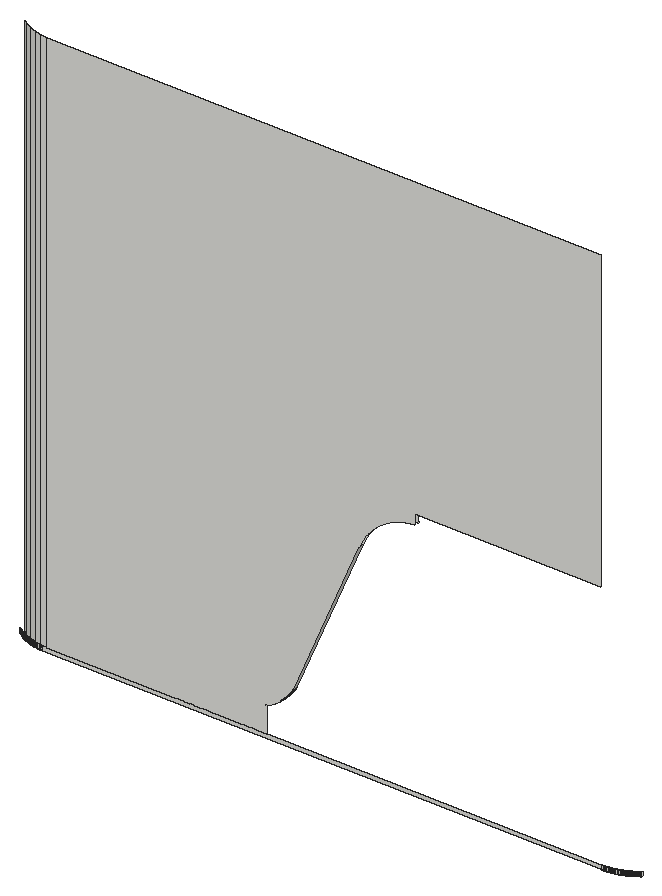
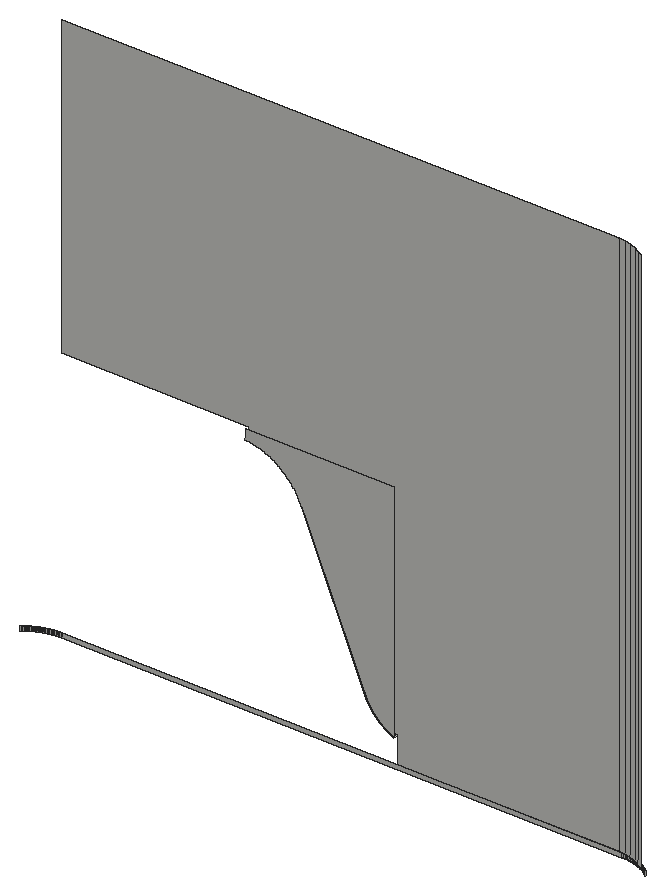
# SketchUp Ruby script. Lengths in inches.
U = 1.inch
M = Sketchup.active_model
def pt(a) = Geom::Point3d.new(a.map { |v| v * U })
def face(e, loops, mat)
  f = e.add_face(loops[0].map { |a| pt(a) })
  loops[1..].each { |l| e.add_face(l.map { |a| pt(a) }).erase! }
  f.material = f.back_material = mat if mat
  f
end
# faces: each face lists its corners as indices into pts; further lists are holes
def faces(e, pts, list, mat = nil) = list.each { |f| face(e, (f[0].is_a?(Array) ? f : [f]).map { |l| l.map { |i| pts[i] } }, mat) }
# xy, xz, yz: faces in a plane at the given z, y or x. An outline is a flat list of corners, or four numbers for a rectangle; further outlines are holes
def ring(l) = l.size == 4 ? [[l[0], l[1]], [l[2], l[1]], [l[2], l[3]], [l[0], l[3]]] : l.each_slice(2).to_a
def flat(e, list, mat, &to3) = list.each { |f| face(e, (f[0].is_a?(Array) ? f : [f]).map { |l| ring(l).map { |u, v| to3.(u, v) } }, mat) }
def xy(e, z, list, mat = nil) = flat(e, list, mat) { |x, y| [x, y, z] }
def xz(e, y, list, mat = nil) = flat(e, list, mat) { |x, z| [x, y, z] }
def yz(e, x, list, mat = nil) = flat(e, list, mat) { |y, z| [x, y, z] }
def lines(e, pts, list) = list.each { |a, b| e.add_line(pt(pts[a]), pt(pts[b])) }
# prism: a flat outline (further loops are holes) pulled along v
def prism(e, loops, v, mat = nil)
  f = face(e, loops, mat); d = Geom::Vector3d.new(v.map { |x| x * U })
  f.pushpull(f.normal.samedirection?(d) ? d.length : -d.length)
end
def box(e, o, s, mat = nil) = prism(e, [[o, [o[0] + s[0], o[1], o[2]], [o[0] + s[0], o[1] + s[1], o[2]], [o[0], o[1] + s[1], o[2]]]], [0, 0, s[2]], mat)
def at(x, y, z, deg = 0) = Geom::Transformation.translation(pt([x, y, z])) * Geom::Transformation.rotation(ORIGIN, Z_AXIS, deg.degrees)
def axes(o, x, y, z) = Geom::Transformation.new([*x, 0, *y, 0, *z, 0, *pt(o).to_a, 1])
def part(name) = M.definitions.add(name)
# library, detail: a bought-in or finely detailed component or shape, given as its bounding box
def library(name, o, s) = part(name).tap { |d| box(d.entities, o, s) }
def detail(e, o, s) = box(e.add_group.entities, o, s)
def put(e, d, t, mat = nil) = e.add_instance(d, t).tap { |i| i.material = mat if mat }
def group(e, t, mat = nil) = e.add_group.tap { |g| g.transformation = t; g.material = mat if mat }.entities
root = M.entities
xz(root,144,[[23.87,130,24.1875,132],[24.1875,130,290.26,132],[290.26,130,290.58,132],[26,132,131,132,131,144.27,130.48,144.04,131,144.28,131.27,144.38,131.36,144.43,131.53,144.5,131.79,144.63,132.04,144.75,132.56,145.01,132.8125,145.14,133.0625,145.28,133.32,145.42,133.57,145.56,133.81,145.7,134.0625,145.85,134.31,146,134.79,146.3,135.04,146.46,135.27,146.61,135.51,146.77,135.75,146.9375,135.98,147.1,136.22,147.27,136.68,147.61,136.9,147.79,137.13,147.97,137.35,148.15,137.58,148.33,137.8,148.51,138.01,148.7,138.23,148.89,138.44,149.08,138.66,149.27,138.87,149.47,139.08,149.66,139.28,149.86,139.49,150.0625,139.6875,150.27,139.89,150.47,140.09,150.68,140.28,150.89,140.48,151.1,140.67,151.32,140.86,151.53,141.05,151.75,141.23,151.97,141.41,152.1875,141.59,152.41,141.77,152.64,141.95,152.86,142.29,153.32,142.46,153.56,142.63,153.79,142.79,154.02,143.27,154.74,143.42,154.98,143.58,155.23,143.73,155.47,175.01,227.16,175.15,227.49,175.3,227.82,175.44,228.14,175.59,228.47,175.74,228.79,175.9,229.11,176.06,229.42,176.22,229.74,176.39,230.05,176.5625,230.36,176.74,230.67,177.1,231.29,177.28,231.59,177.66,232.19,177.86,232.49,178.26,233.07,178.68,233.65,178.89,233.9375,179.1,234.22,179.32,234.5,179.55,234.78,179.77,235.05,180,235.33,180.23,235.6,180.46,235.86,180.7,236.13,180.94,236.39,181.1875,236.65,181.43,236.9,181.68,237.16,181.93,237.41,182.19,237.66,182.97,238.38,183.24,238.62,184.05,239.31,184.89,239.97,185.18,240.18,185.46,240.39,185.75,240.6,186.04,240.8,186.34,241,186.63,241.2,187.23,241.58,187.54,241.77,187.84,241.95,188.46,242.31,189.08,242.65,189.4,242.8125,189.71,242.97,190.35,243.29,190.67,243.4375,191,243.58,191.32,243.73,191.65,243.87,192.97,244.39,193.31,244.51,193.64,244.625,193.98,244.74,194.32,244.85,195.34,245.15,195.68,245.24,196.03,245.33,196.375,245.42,196.72,245.5,197.07,245.58,197.42,245.65,197.76,245.72,198.11,245.78,198.46,245.85,198.81,245.9,199.17,245.96,199.52,246.01,200.22,246.09,200.58,246.13,200.93,246.16,201.29,246.19,201.64,246.22,201.56,248,201.56,251,290.45,251,290.45,392.81,26,392.81],[130.48,144.04,131,144.27,131,144.28]])
xz(root,146,[[131,144.28,131,251,201.56,251,201.56,248,201.64,246.22,201.29,246.19,200.93,246.16,200.58,246.13,200.22,246.09,199.52,246.01,199.17,245.96,198.81,245.9,198.46,245.85,198.11,245.78,197.76,245.72,197.42,245.65,197.07,245.58,196.72,245.5,196.375,245.42,196.03,245.33,195.68,245.24,195.34,245.15,194.32,244.85,193.98,244.74,193.64,244.625,193.31,244.51,192.97,244.39,191.65,243.87,191.32,243.73,191,243.58,190.67,243.4375,190.35,243.29,189.71,242.97,189.4,242.8125,189.08,242.65,188.46,242.31,187.84,241.95,187.54,241.77,187.23,241.58,186.63,241.2,186.34,241,186.04,240.8,185.75,240.6,185.46,240.39,185.18,240.18,184.89,239.97,184.05,239.31,183.24,238.62,182.97,238.38,182.19,237.66,181.93,237.41,181.68,237.16,181.43,236.9,181.1875,236.65,180.94,236.39,180.7,236.13,180.46,235.86,180.23,235.6,180,235.33,179.77,235.05,179.55,234.78,179.32,234.5,179.1,234.22,178.89,233.9375,178.68,233.65,178.26,233.07,177.86,232.49,177.66,232.19,177.28,231.59,177.1,231.29,176.74,230.67,176.5625,230.36,176.39,230.05,176.22,229.74,176.06,229.42,175.9,229.11,175.74,228.79,175.59,228.47,175.44,228.14,175.3,227.82,175.15,227.49,175.01,227.16,143.73,155.47,143.58,155.23,143.42,154.98,143.27,154.74,142.79,154.02,142.63,153.79,142.46,153.56,142.29,153.32,141.95,152.86,141.77,152.64,141.59,152.41,141.41,152.1875,141.23,151.97,141.05,151.75,140.86,151.53,140.67,151.32,140.48,151.1,140.28,150.89,140.09,150.68,139.89,150.47,139.6875,150.27,139.49,150.0625,139.28,149.86,139.08,149.66,138.87,149.47,138.66,149.27,138.44,149.08,138.23,148.89,138.01,148.7,137.8,148.51,137.58,148.33,137.35,148.15,137.13,147.97,136.9,147.79,136.68,147.61,136.22,147.27,135.98,147.1,135.75,146.9375,135.51,146.77,135.27,146.61,135.04,146.46,134.79,146.3,134.31,146,134.0625,145.85,133.81,145.7,133.57,145.56,133.32,145.42,133.0625,145.28,132.8125,145.14,132.56,145.01,132.04,144.75,131.79,144.63,131.53,144.5,131.36,144.43,131.27,144.38]])
p = [[22.61,144.05,130],[22.92,144.03,130],[22.92,144.03,132],[22.61,144.05,132],[23.24,144.02,130],[23.24,144.02,132],
  [23.56,144.01,130],[23.56,144.01,132],[23.87,144,130],[23.87,144,132],[290.58,144,130],[290.9,144.01,130],
  [290.9,144.01,132],[290.58,144,132],[291.21,144.02,130],[291.21,144.02,132],[291.53,144.03,130],[291.53,144.03,132],
  [291.85,144.05,130],[291.85,144.05,132],[21.35,144.17,130],[21.66,144.13,130],[21.66,144.13,132],[21.35,144.17,132],
  [21.98,144.1,130],[21.98,144.1,132],[22.29,144.07,130],[22.29,144.07,132],[292.16,144.07,130],[292.16,144.07,132],
  [292.48,144.1,130],[292.48,144.1,132],[292.79,144.13,130],[292.79,144.13,132],[293.11,144.17,130],[293.11,144.17,132],
  [20.4,144.3,130],[20.72,144.25,130],[20.72,144.25,132],[20.4,144.3,132],[21.03,144.21,130],[21.03,144.21,132],
  [293.42,144.21,130],[293.42,144.21,132],[293.74,144.25,130],[293.74,144.25,132],[294.05,144.3,130],[294.05,144.3,132],
  [19.78,144.4,130],[20.09,144.35,130],[20.09,144.35,132],[19.78,144.4,132],[294.36,144.35,130],[294.36,144.35,132],
  [294.67,144.4,130],[294.67,144.4,132],[19.47,144.46,130],[19.47,144.46,132],[294.98,144.46,130],[294.98,144.46,132],
  [18.85,144.59,130],[19.16,144.52,130],[19.16,144.52,132],[18.85,144.59,132],[295.29,144.52,130],[295.29,144.52,132],
  [295.6,144.59,130],[295.6,144.59,132],[18.54,144.66,130],[18.54,144.66,132],[295.91,144.66,130],[295.91,144.66,132],
  [17.93,144.82,130],[18.23,144.74,130],[18.23,144.74,132],[17.93,144.82,132],[296.22,144.74,130],[296.22,144.74,132],
  [296.53,144.82,130],[296.53,144.82,132],[17.62,144.9,130],[17.62,144.9,132],[296.83,144.9,130],[296.83,144.9,132],
  [17.32,144.99,130],[17.32,144.99,132],[297.13,144.99,130],[297.13,144.99,132],[17.02,145.08,130],[17.02,145.08,132],
  [297.4375,145.08,130],[297.4375,145.08,132],[16.71,145.17,130],[16.71,145.17,132],[297.74,145.17,130],[297.74,145.17,132],
  [16.41,145.27,130],[16.41,145.27,132],[298.04,145.27,130],[298.04,145.27,132],[16.11,145.375,130],[16.11,145.375,132],
  [298.34,145.375,130],[298.34,145.375,132],[15.82,145.48,130],[15.82,145.48,132],[298.64,145.48,130],[298.64,145.48,132],
  [15.52,145.59,130],[15.52,145.59,132],[298.93,145.59,130],[298.93,145.59,132],[15.23,145.71,130],[15.23,145.71,132],
  [299.23,145.71,130],[299.23,145.71,132],[14.93,145.83,130],[14.93,145.83,132],[299.52,145.83,130],[299.52,145.83,132],
  [14.64,145.95,130],[14.64,145.95,132],[299.8125,145.95,130],[299.8125,145.95,132],[14.35,146.07,130],[14.35,146.07,132],
  [300.1,146.07,130],[300.1,146.07,132],[14.0625,146.2,130],[14.0625,146.2,132],[300.39,146.2,130],[300.39,146.2,132],
  [13.78,146.34,130],[13.78,146.34,132],[300.68,146.34,130],[300.68,146.34,132],[13.49,146.48,130],[13.49,146.48,132],
  [300.96,146.48,130],[300.96,146.48,132],[13.21,146.62,130],[13.21,146.62,132],[301.25,146.62,130],[301.25,146.62,132],
  [12.93,146.76,130],[12.93,146.76,132],[301.53,146.76,130],[301.53,146.76,132],[12.65,146.91,130],[12.65,146.91,132],
  [301.81,146.91,130],[301.81,146.91,132],[12.37,147.06,130],[12.37,147.06,132],[302.08,147.06,130],[302.08,147.06,132],
  [12.09,147.22,130],[12.09,147.22,132],[302.36,147.22,130],[302.36,147.22,132],[11.82,147.375,130],[11.82,147.375,132],
  [302.63,147.375,130],[302.63,147.375,132],[11.55,147.54,130],[11.55,147.54,132],[302.9,147.54,130],[302.9,147.54,132],
  [11.28,147.7,130],[11.28,147.7,132],[303.17,147.7,130],[303.17,147.7,132],[11.01,147.87,130],[11.01,147.87,132],
  [303.4375,147.87,130],[303.4375,147.87,132],[10.75,148.04,130],[10.75,148.04,132],[303.7,148.04,130],[303.7,148.04,132],
  [10.49,148.22,130],[10.49,148.22,132],[303.97,148.22,130],[303.97,148.22,132],[10.23,148.4,130],[10.23,148.4,132],
  [304.23,148.4,130],[304.23,148.4,132],[9.97,148.58,130],[9.97,148.58,132],[304.48,148.58,130],[304.48,148.58,132],
  [9.72,148.77,130],[9.72,148.77,132],[304.74,148.77,130],[304.74,148.77,132],[9.46,148.96,130],[9.46,148.96,132],
  [304.99,148.96,130],[304.99,148.96,132],[9.21,149.15,130],[9.21,149.15,132],[305.24,149.15,130],[305.24,149.15,132],
  [8.97,149.35,130],[8.97,149.35,132],[305.49,149.35,130],[305.49,149.35,132],[8.72,149.55,130],[8.72,149.55,132],
  [305.73,149.55,130],[305.73,149.55,132],[22.87,144.21,132],[26,144,132],[26,144,392.81],[22.87,144.21,392.81],
  [19.79,144.82,132],[19.79,144.82,392.81],[16.82,145.83,132],[16.82,145.83,392.81],[14,147.22,132],[14,147.22,392.81],
  [11.39,148.96,132],[11.39,148.96,392.81],[131.27,144,144.38],[131,144,144.28],[131,146,144.28],[131.27,146,144.38],
  [131.36,144,144.43],[131.36,146,144.43],[131.53,144,144.5],[131.53,146,144.5],[131.79,144,144.63],[131.79,146,144.63],
  [132.04,144,144.75],[132.04,146,144.75],[132.3,144,144.88],[132.3,146,144.88],[132.56,144,145.01],[132.56,146,145.01],
  [132.8125,144,145.14],[132.8125,146,145.14],[133.0625,144,145.28],[133.0625,146,145.28],[133.32,144,145.42],[133.32,146,145.42],
  [133.57,144,145.56],[133.57,146,145.56],[133.81,144,145.7],[133.81,146,145.7],[134.0625,144,145.85],[134.0625,146,145.85],
  [134.31,144,146],[134.31,146,146],[134.55,144,146.15],[134.55,146,146.15],[134.79,144,146.3],[134.79,146,146.3],
  [135.04,144,146.46],[135.04,146,146.46],[135.27,144,146.61],[135.27,146,146.61],[135.51,144,146.77],[135.51,146,146.77],
  [135.75,144,146.9375],[135.75,146,146.9375],[135.98,144,147.1],[135.98,146,147.1],[136.22,144,147.27],[136.22,146,147.27],
  [136.45,144,147.44],[136.45,146,147.44],[136.68,144,147.61],[136.68,146,147.61],[136.9,144,147.79],[136.9,146,147.79],
  [137.13,144,147.97],[137.13,146,147.97],[137.35,144,148.15],[137.35,146,148.15],[137.58,144,148.33],[137.58,146,148.33],
  [137.8,144,148.51],[137.8,146,148.51],[138.01,144,148.7],[138.01,146,148.7],[138.23,144,148.89],[138.23,146,148.89],
  [138.44,144,149.08],[138.44,146,149.08],[138.66,144,149.27],[138.66,146,149.27],[138.87,144,149.47],[138.87,146,149.47],
  [139.08,144,149.66],[139.08,146,149.66],[139.28,144,149.86],[139.28,146,149.86],[139.49,144,150.0625],[139.49,146,150.0625],
  [139.6875,144,150.27],[139.6875,146,150.27],[139.89,144,150.47],[139.89,146,150.47],[140.09,144,150.68],[140.09,146,150.68],
  [140.28,144,150.89],[140.28,146,150.89],[140.48,144,151.1],[140.48,146,151.1],[140.67,144,151.32],[140.67,146,151.32],
  [140.86,144,151.53],[140.86,146,151.53],[141.05,144,151.75],[141.05,146,151.75],[141.23,144,151.97],[141.23,146,151.97],
  [141.41,144,152.1875],[141.41,146,152.1875],[141.59,144,152.41],[141.59,146,152.41],[141.77,144,152.64],[141.77,146,152.64],
  [141.95,144,152.86],[141.95,146,152.86],[142.12,144,153.09],[142.12,146,153.09],[142.29,144,153.32],[142.29,146,153.32],
  [142.46,144,153.56],[142.46,146,153.56],[142.63,144,153.79],[142.63,146,153.79],[142.79,144,154.02],[142.79,146,154.02],
  [142.95,144,154.26],[142.95,146,154.26],[143.11,144,154.5],[143.11,146,154.5],[143.27,144,154.74],[143.27,146,154.74],
  [143.42,144,154.98],[143.42,146,154.98],[143.58,144,155.23],[143.58,146,155.23],[143.73,144,155.47],[143.73,146,155.47],
  [175.01,144,227.16],[175.01,146,227.16],[131.36,144,144.42]]
faces(root,p,[[0,1,2,3],[1,4,5,2],[4,6,7,5],[6,8,9,7],[10,11,12,13],[11,14,15,12],[14,16,17,15],[16,18,19,17],
  [20,21,22,23],[21,24,25,22],[24,26,27,25],[26,0,3,27],[18,28,29,19],[28,30,31,29],[30,32,33,31],[32,34,35,33],
  [36,37,38,39],[37,40,41,38],[40,20,23,41],[34,42,43,35],[42,44,45,43],[44,46,47,45],[48,49,50,51],[49,36,39,50],
  [46,52,53,47],[52,54,55,53],[56,48,51,57],[54,58,59,55],[60,61,62,63],[61,56,57,62],[58,64,65,59],[64,66,67,65],
  [68,60,63,69],[66,70,71,67],[72,73,74,75],[73,68,69,74],[70,76,77,71],[76,78,79,77],[80,72,75,81],[78,82,83,79],
  [84,80,81,85],[82,86,87,83],[88,84,85,89],[86,90,91,87],[92,88,89,93],[90,94,95,91],[96,92,93,97],[94,98,99,95],
  [100,96,97,101],[98,102,103,99],[104,100,101,105],[102,106,107,103],[108,104,105,109],[106,110,111,107],[112,108,109,113],[110,114,115,111],
  [116,112,113,117],[114,118,119,115],[120,116,117,121],[118,122,123,119],[124,120,121,125],[122,126,127,123],[128,124,125,129],[126,130,131,127],
  [132,128,129,133],[130,134,135,131],[136,132,133,137],[134,138,139,135],[140,136,137,141],[138,142,143,139],[144,140,141,145],[142,146,147,143],
  [148,144,145,149],[146,150,151,147],[152,148,149,153],[150,154,155,151],[156,152,153,157],[154,158,159,155],[160,156,157,161],[158,162,163,159],
  [164,160,161,165],[162,166,167,163],[168,164,165,169],[166,170,171,167],[172,168,169,173],[170,174,175,171],[176,172,173,177],[174,178,179,175],
  [180,176,177,181],[178,182,183,179],[184,180,181,185],[182,186,187,183],[188,184,185,189],[186,190,191,187],[192,188,189,193],[190,194,195,191],
  [196,192,193,197],[194,198,199,195],[200,196,197,201],[198,202,203,199],[204,200,201,205],[202,206,207,203],[208,204,205,209],[206,210,211,207],
  [212,213,214,215],[216,212,215,217],[218,216,217,219],[220,218,219,221],[222,220,221,223],[224,225,226,227],[228,224,227,229],[230,228,229,231],
  [232,230,231,233],[234,232,233,235],[236,234,235,237],[238,236,237,239],[240,238,239,241],[242,240,241,243],[244,242,243,245],[246,244,245,247],
  [248,246,247,249],[250,248,249,251],[252,250,251,253],[254,252,253,255],[256,254,255,257],[258,256,257,259],[260,258,259,261],[262,260,261,263],
  [264,262,263,265],[266,264,265,267],[268,266,267,269],[270,268,269,271],[272,270,271,273],[274,272,273,275],[276,274,275,277],[278,276,277,279],
  [280,278,279,281],[282,280,281,283],[284,282,283,285],[286,284,285,287],[288,286,287,289],[290,288,289,291],[292,290,291,293],[294,292,293,295],
  [296,294,295,297],[298,296,297,299],[300,298,299,301],[302,300,301,303],[304,302,303,305],[306,304,305,307],[308,306,307,309],[310,308,309,311],
  [312,310,311,313],[314,312,313,315],[316,314,315,317],[318,316,317,319],[320,318,319,321],[322,320,321,323],[324,322,323,325],[326,324,325,327],
  [328,326,327,329],[330,328,329,331],[332,330,331,333],[334,332,333,335],[336,334,335,337],[338,336,337,339],[340,338,339,341],[342,340,341,343],
  [344,342,343,345],[346,344,345,347],[348,346,347,349]])
lines(root,p,[[350,228]])
